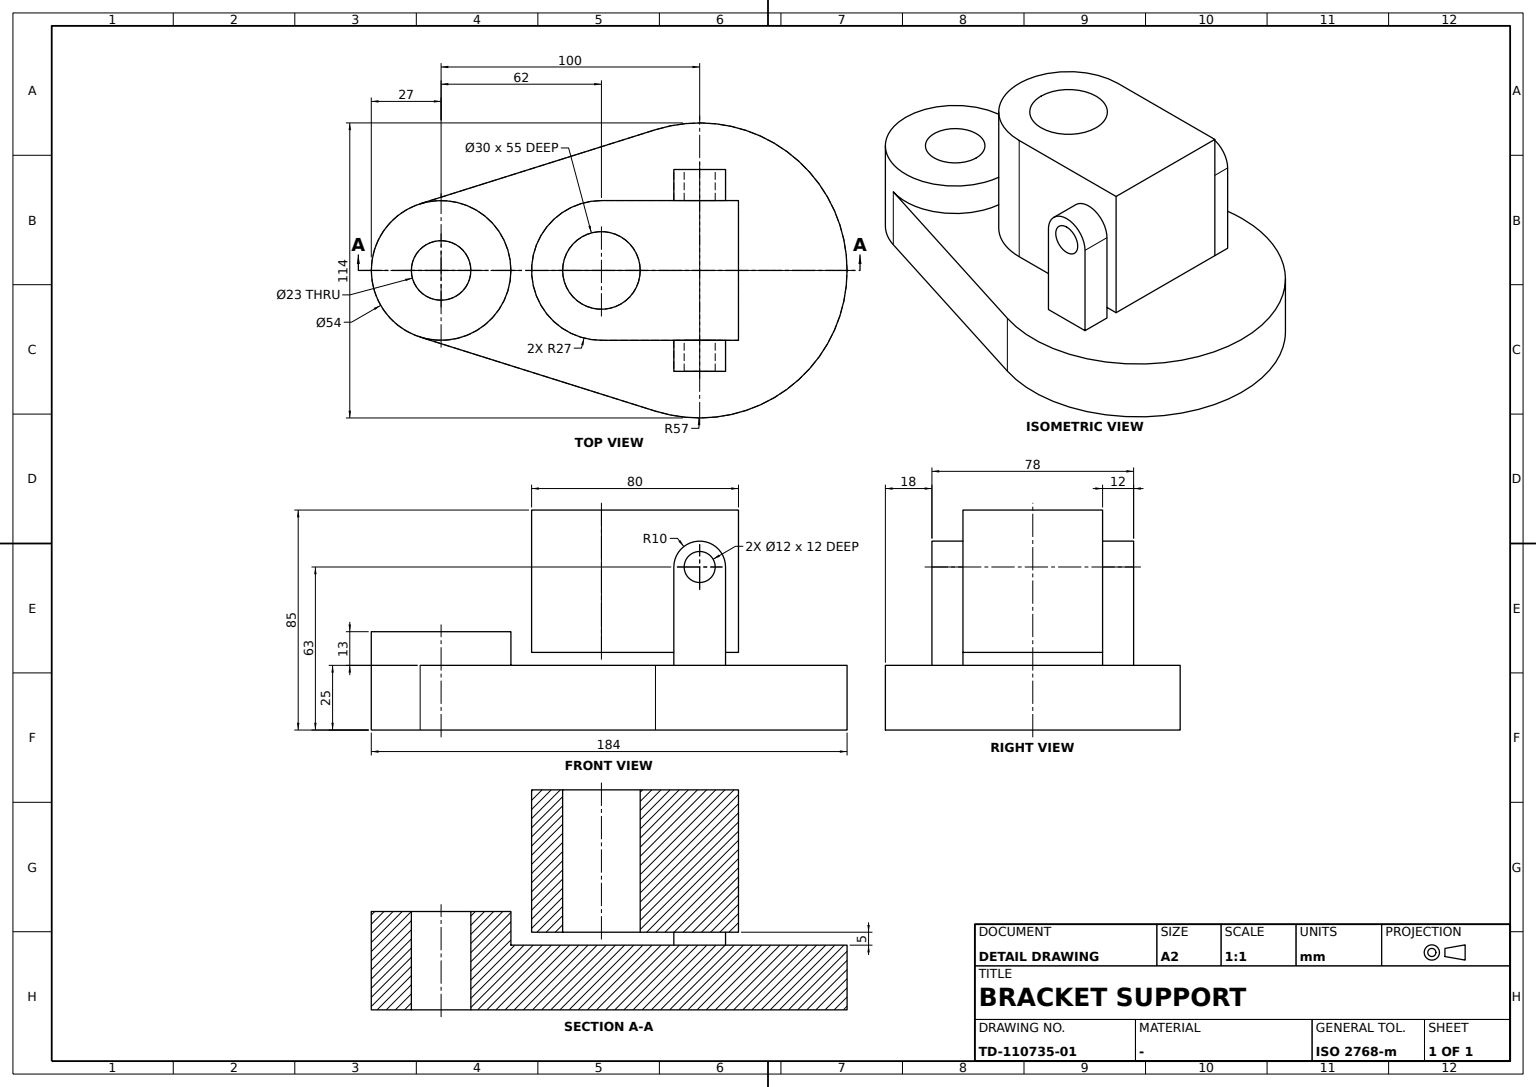
ISO-10303-21;
HEADER;
FILE_DESCRIPTION((''),'2;1');
FILE_NAME('','',(''),(''),'','','');
FILE_SCHEMA(('AUTOMOTIVE_DESIGN'));
ENDSEC;
DATA;
#1=APPLICATION_CONTEXT('');
#2=PRODUCT_CONTEXT('',#1,'mechanical');
#3=PRODUCT('','','',(#2));
#4=PRODUCT_DEFINITION_FORMATION('','',#3);
#5=PRODUCT_DEFINITION_CONTEXT('',#1,'design');
#6=PRODUCT_DEFINITION('','',#4,#5);
#7=PRODUCT_DEFINITION_SHAPE('','',#6);
#8=(LENGTH_UNIT()NAMED_UNIT(*)SI_UNIT(.MILLI.,.METRE.));
#9=(NAMED_UNIT(*)PLANE_ANGLE_UNIT()SI_UNIT($,.RADIAN.));
#10=(NAMED_UNIT(*)SI_UNIT($,.STERADIAN.)SOLID_ANGLE_UNIT());
#11=UNCERTAINTY_MEASURE_WITH_UNIT(LENGTH_MEASURE(0.005),#8,'distance_accuracy_value','');
#12=(GEOMETRIC_REPRESENTATION_CONTEXT(3)GLOBAL_UNCERTAINTY_ASSIGNED_CONTEXT((#11))GLOBAL_UNIT_ASSIGNED_CONTEXT((#8,#9,#10))REPRESENTATION_CONTEXT('',''));
#13=CARTESIAN_POINT('',(100.,27.,69.));
#14=VERTEX_POINT('',#13);
#15=CARTESIAN_POINT('',(100.,27.,63.));
#16=DIRECTION('',(0.,1.,0.));
#17=DIRECTION('',(0.,0.,1.));
#18=AXIS2_PLACEMENT_3D('',#15,#16,#17);
#19=CIRCLE('',#18,6.);
#20=EDGE_CURVE('',#14,#14,#19,.T.);
#21=ORIENTED_EDGE('',*,*,#20,.F.);
#22=EDGE_LOOP('',(#21));
#23=FACE_BOUND('',#22,.T.);
#24=CARTESIAN_POINT('',(100.,39.,57.));
#25=VERTEX_POINT('',#24);
#26=CARTESIAN_POINT('',(100.,39.,63.));
#27=DIRECTION('',(0.,-1.,0.));
#28=DIRECTION('',(0.,0.,-1.));
#29=AXIS2_PLACEMENT_3D('',#26,#27,#28);
#30=CIRCLE('',#29,6.);
#31=EDGE_CURVE('',#25,#25,#30,.F.);
#32=ORIENTED_EDGE('',*,*,#31,.T.);
#33=EDGE_LOOP('',(#32));
#34=FACE_BOUND('',#33,.T.);
#35=CARTESIAN_POINT('',(100.,-9.66,63.));
#36=DIRECTION('',(-1.,0.,0.));
#37=AXIS2_PLACEMENT_3D('',#35,#16,#36);
#38=CYLINDRICAL_SURFACE('',#37,6.);
#39=ADVANCED_FACE('',(#23,#34),#38,.F.);
#40=CARTESIAN_POINT('',(115.,-27.,85.));
#41=VERTEX_POINT('',#40);
#42=CARTESIAN_POINT('',(115.,27.,85.));
#43=VERTEX_POINT('',#42);
#44=CARTESIAN_POINT('',(115.,0.,85.));
#45=VECTOR('',#16,1000.);
#46=LINE('',#44,#45);
#47=EDGE_CURVE('',#41,#43,#46,.T.);
#48=ORIENTED_EDGE('',*,*,#47,.F.);
#49=CARTESIAN_POINT('',(115.,-27.,30.));
#50=VERTEX_POINT('',#49);
#51=CARTESIAN_POINT('',(115.,-27.,25.));
#52=VECTOR('',#17,1000.);
#53=LINE('',#51,#52);
#54=EDGE_CURVE('',#50,#41,#53,.T.);
#55=ORIENTED_EDGE('',*,*,#54,.F.);
#56=CARTESIAN_POINT('',(115.,27.,30.));
#57=VERTEX_POINT('',#56);
#58=CARTESIAN_POINT('',(115.,0.,30.));
#59=LINE('',#58,#45);
#60=EDGE_CURVE('',#50,#57,#59,.T.);
#61=ORIENTED_EDGE('',*,*,#60,.T.);
#62=CARTESIAN_POINT('',(115.,27.,25.));
#63=LINE('',#62,#52);
#64=EDGE_CURVE('',#57,#43,#63,.T.);
#65=ORIENTED_EDGE('',*,*,#64,.T.);
#66=EDGE_LOOP('',(#48,#55,#61,#65));
#67=FACE_BOUND('',#66,.T.);
#68=AXIS2_PLACEMENT_3D('',#58,#36,#17);
#69=PLANE('',#68);
#70=ADVANCED_FACE('',(#67),#69,.F.);
#71=CARTESIAN_POINT('',(100.,-39.,57.));
#72=VERTEX_POINT('',#71);
#73=CARTESIAN_POINT('',(100.,-39.,63.));
#74=AXIS2_PLACEMENT_3D('',#73,#27,#28);
#75=CIRCLE('',#74,6.);
#76=EDGE_CURVE('',#72,#72,#75,.T.);
#77=ORIENTED_EDGE('',*,*,#76,.F.);
#78=EDGE_LOOP('',(#77));
#79=FACE_BOUND('',#78,.T.);
#80=CARTESIAN_POINT('',(90.,-39.,25.));
#81=VERTEX_POINT('',#80);
#82=CARTESIAN_POINT('',(90.,-39.,63.));
#83=VERTEX_POINT('',#82);
#84=LINE('',#80,#52);
#85=EDGE_CURVE('',#81,#83,#84,.T.);
#86=ORIENTED_EDGE('',*,*,#85,.F.);
#87=CARTESIAN_POINT('',(110.,-39.,25.));
#88=VERTEX_POINT('',#87);
#89=CARTESIAN_POINT('',(0.,-39.,25.));
#90=DIRECTION('',(1.,0.,0.));
#91=VECTOR('',#90,1000.);
#92=LINE('',#89,#91);
#93=EDGE_CURVE('',#81,#88,#92,.T.);
#94=ORIENTED_EDGE('',*,*,#93,.T.);
#95=CARTESIAN_POINT('',(110.,-39.,62.999996));
#96=VERTEX_POINT('',#95);
#97=LINE('',#87,#52);
#98=EDGE_CURVE('',#88,#96,#97,.T.);
#99=ORIENTED_EDGE('',*,*,#98,.T.);
#100=CIRCLE('',#74,10.);
#101=EDGE_CURVE('',#96,#83,#100,.T.);
#102=ORIENTED_EDGE('',*,*,#101,.T.);
#103=EDGE_LOOP('',(#86,#94,#99,#102));
#104=FACE_BOUND('',#103,.T.);
#105=AXIS2_PLACEMENT_3D('',#80,#27,#90);
#106=PLANE('',#105);
#107=ADVANCED_FACE('',(#79,#104),#106,.T.);
#108=CARTESIAN_POINT('',(90.,-27.,25.));
#109=VERTEX_POINT('',#108);
#110=CARTESIAN_POINT('',(90.,-27.,30.));
#111=VERTEX_POINT('',#110);
#112=LINE('',#108,#52);
#113=EDGE_CURVE('',#109,#111,#112,.T.);
#114=ORIENTED_EDGE('',*,*,#113,.T.);
#115=CARTESIAN_POINT('',(110.,-27.,30.));
#116=VERTEX_POINT('',#115);
#117=LINE('',#115,#91);
#118=EDGE_CURVE('',#111,#116,#117,.T.);
#119=ORIENTED_EDGE('',*,*,#118,.T.);
#120=CARTESIAN_POINT('',(110.,-27.,25.));
#121=VERTEX_POINT('',#120);
#122=LINE('',#120,#52);
#123=EDGE_CURVE('',#121,#116,#122,.T.);
#124=ORIENTED_EDGE('',*,*,#123,.F.);
#125=CARTESIAN_POINT('',(0.,-27.,25.));
#126=VECTOR('',#36,1000.);
#127=LINE('',#125,#126);
#128=EDGE_CURVE('',#121,#109,#127,.T.);
#129=ORIENTED_EDGE('',*,*,#128,.T.);
#130=EDGE_LOOP('',(#114,#119,#124,#129));
#131=FACE_BOUND('',#130,.T.);
#132=AXIS2_PLACEMENT_3D('',#120,#16,#36);
#133=PLANE('',#132);
#134=ADVANCED_FACE('',(#131),#133,.T.);
#135=CARTESIAN_POINT('',(62.,27.,85.));
#136=VERTEX_POINT('',#135);
#137=CARTESIAN_POINT('',(62.,27.,30.));
#138=VERTEX_POINT('',#137);
#139=CARTESIAN_POINT('',(62.,27.,57.5));
#140=VECTOR('',#28,1000.);
#141=LINE('',#139,#140);
#142=EDGE_CURVE('',#136,#138,#141,.T.);
#143=ORIENTED_EDGE('',*,*,#142,.T.);
#144=CARTESIAN_POINT('',(62.,-27.,30.));
#145=VERTEX_POINT('',#144);
#146=CARTESIAN_POINT('',(62.,0.,30.));
#147=AXIS2_PLACEMENT_3D('',#146,#17,#90);
#148=CIRCLE('',#147,27.);
#149=EDGE_CURVE('',#138,#145,#148,.T.);
#150=ORIENTED_EDGE('',*,*,#149,.T.);
#151=CARTESIAN_POINT('',(62.,-27.,85.));
#152=VERTEX_POINT('',#151);
#153=CARTESIAN_POINT('',(62.,-27.,57.5));
#154=LINE('',#153,#140);
#155=EDGE_CURVE('',#152,#145,#154,.T.);
#156=ORIENTED_EDGE('',*,*,#155,.F.);
#157=CARTESIAN_POINT('',(62.,0.,85.));
#158=AXIS2_PLACEMENT_3D('',#157,#28,#36);
#159=CIRCLE('',#158,27.);
#160=EDGE_CURVE('',#152,#136,#159,.T.);
#161=ORIENTED_EDGE('',*,*,#160,.T.);
#162=EDGE_LOOP('',(#143,#150,#156,#161));
#163=FACE_BOUND('',#162,.T.);
#164=CARTESIAN_POINT('',(62.,0.,57.5));
#165=AXIS2_PLACEMENT_3D('',#164,#28,#27);
#166=CYLINDRICAL_SURFACE('',#165,27.);
#167=ADVANCED_FACE('',(#163),#166,.T.);
#168=CARTESIAN_POINT('',(47.,0.,85.));
#169=VERTEX_POINT('',#168);
#170=CIRCLE('',#158,15.);
#171=EDGE_CURVE('',#169,#169,#170,.T.);
#172=ORIENTED_EDGE('',*,*,#171,.T.);
#173=EDGE_LOOP('',(#172));
#174=FACE_BOUND('',#173,.T.);
#175=CARTESIAN_POINT('',(110.,-27.,85.));
#176=LINE('',#175,#126);
#177=EDGE_CURVE('',#41,#152,#176,.T.);
#178=ORIENTED_EDGE('',*,*,#177,.F.);
#179=ORIENTED_EDGE('',*,*,#47,.T.);
#180=CARTESIAN_POINT('',(110.,27.,85.));
#181=LINE('',#180,#126);
#182=EDGE_CURVE('',#43,#136,#181,.T.);
#183=ORIENTED_EDGE('',*,*,#182,.T.);
#184=ORIENTED_EDGE('',*,*,#160,.F.);
#185=EDGE_LOOP('',(#178,#179,#183,#184));
#186=FACE_BOUND('',#185,.T.);
#187=AXIS2_PLACEMENT_3D('',#44,#28,#36);
#188=PLANE('',#187);
#189=ADVANCED_FACE('',(#174,#186),#188,.F.);
#190=CARTESIAN_POINT('',(100.,-27.,69.));
#191=VERTEX_POINT('',#190);
#192=CARTESIAN_POINT('',(100.,-27.,63.));
#193=AXIS2_PLACEMENT_3D('',#192,#16,#17);
#194=CIRCLE('',#193,6.);
#195=EDGE_CURVE('',#191,#191,#194,.T.);
#196=ORIENTED_EDGE('',*,*,#195,.F.);
#197=EDGE_LOOP('',(#196));
#198=FACE_BOUND('',#197,.T.);
#199=ADVANCED_FACE('',(#198),#133,.F.);
#200=CARTESIAN_POINT('',(90.,27.,25.));
#201=VERTEX_POINT('',#200);
#202=CARTESIAN_POINT('',(90.,39.,25.));
#203=VERTEX_POINT('',#202);
#204=CARTESIAN_POINT('',(90.,0.,25.));
#205=LINE('',#204,#45);
#206=EDGE_CURVE('',#201,#203,#205,.T.);
#207=ORIENTED_EDGE('',*,*,#206,.F.);
#208=CARTESIAN_POINT('',(90.,27.,30.));
#209=VERTEX_POINT('',#208);
#210=LINE('',#200,#52);
#211=EDGE_CURVE('',#201,#209,#210,.T.);
#212=ORIENTED_EDGE('',*,*,#211,.T.);
#213=CARTESIAN_POINT('',(90.,27.,63.));
#214=VERTEX_POINT('',#213);
#215=EDGE_CURVE('',#209,#214,#210,.T.);
#216=ORIENTED_EDGE('',*,*,#215,.T.);
#217=CARTESIAN_POINT('',(90.,39.,63.));
#218=VERTEX_POINT('',#217);
#219=CARTESIAN_POINT('',(90.,33.,63.));
#220=LINE('',#219,#45);
#221=EDGE_CURVE('',#214,#218,#220,.T.);
#222=ORIENTED_EDGE('',*,*,#221,.T.);
#223=LINE('',#202,#52);
#224=EDGE_CURVE('',#203,#218,#223,.T.);
#225=ORIENTED_EDGE('',*,*,#224,.F.);
#226=EDGE_LOOP('',(#207,#212,#216,#222,#225));
#227=FACE_BOUND('',#226,.T.);
#228=AXIS2_PLACEMENT_3D('',#200,#90,#16);
#229=PLANE('',#228);
#230=ADVANCED_FACE('',(#227),#229,.F.);
#231=CARTESIAN_POINT('',(110.,27.,25.));
#232=VERTEX_POINT('',#231);
#233=CARTESIAN_POINT('',(110.,27.,30.));
#234=VERTEX_POINT('',#233);
#235=LINE('',#231,#52);
#236=EDGE_CURVE('',#232,#234,#235,.T.);
#237=ORIENTED_EDGE('',*,*,#236,.T.);
#238=LINE('',#233,#91);
#239=EDGE_CURVE('',#209,#234,#238,.T.);
#240=ORIENTED_EDGE('',*,*,#239,.F.);
#241=ORIENTED_EDGE('',*,*,#211,.F.);
#242=CARTESIAN_POINT('',(0.,27.,25.));
#243=LINE('',#242,#126);
#244=EDGE_CURVE('',#232,#201,#243,.T.);
#245=ORIENTED_EDGE('',*,*,#244,.F.);
#246=EDGE_LOOP('',(#237,#240,#241,#245));
#247=FACE_BOUND('',#246,.T.);
#248=AXIS2_PLACEMENT_3D('',#231,#16,#36);
#249=PLANE('',#248);
#250=ADVANCED_FACE('',(#247),#249,.F.);
#251=CARTESIAN_POINT('',(82.9,-54.374534,25.));
#252=VERTEX_POINT('',#251);
#253=CARTESIAN_POINT('',(82.9,54.374534,25.));
#254=VERTEX_POINT('',#253);
#255=CARTESIAN_POINT('',(100.,0.,25.));
#256=AXIS2_PLACEMENT_3D('',#255,#17,#90);
#257=CIRCLE('',#256,57.);
#258=EDGE_CURVE('',#252,#254,#257,.T.);
#259=ORIENTED_EDGE('',*,*,#258,.F.);
#260=CARTESIAN_POINT('',(82.9,-54.374534,0.));
#261=VERTEX_POINT('',#260);
#262=CARTESIAN_POINT('',(82.9,-54.374534,12.5));
#263=LINE('',#262,#52);
#264=EDGE_CURVE('',#261,#252,#263,.T.);
#265=ORIENTED_EDGE('',*,*,#264,.F.);
#266=CARTESIAN_POINT('',(82.9,54.374534,0.));
#267=VERTEX_POINT('',#266);
#268=CARTESIAN_POINT('',(100.,0.,0.));
#269=AXIS2_PLACEMENT_3D('',#268,#17,#90);
#270=CIRCLE('',#269,57.);
#271=EDGE_CURVE('',#261,#267,#270,.T.);
#272=ORIENTED_EDGE('',*,*,#271,.T.);
#273=CARTESIAN_POINT('',(82.9,54.374534,12.5));
#274=LINE('',#273,#52);
#275=EDGE_CURVE('',#267,#254,#274,.T.);
#276=ORIENTED_EDGE('',*,*,#275,.T.);
#277=EDGE_LOOP('',(#259,#265,#272,#276));
#278=FACE_BOUND('',#277,.T.);
#279=CARTESIAN_POINT('',(100.,0.,12.5));
#280=AXIS2_PLACEMENT_3D('',#279,#17,#90);
#281=CYLINDRICAL_SURFACE('',#280,57.);
#282=ADVANCED_FACE('',(#278),#281,.T.);
#283=CARTESIAN_POINT('',(90.,-27.,62.999996));
#284=VERTEX_POINT('',#283);
#285=CARTESIAN_POINT('',(110.,-27.,63.));
#286=VERTEX_POINT('',#285);
#287=CIRCLE('',#193,10.);
#288=EDGE_CURVE('',#284,#286,#287,.T.);
#289=ORIENTED_EDGE('',*,*,#288,.F.);
#290=EDGE_CURVE('',#83,#284,#220,.T.);
#291=ORIENTED_EDGE('',*,*,#290,.F.);
#292=ORIENTED_EDGE('',*,*,#101,.F.);
#293=CARTESIAN_POINT('',(110.,33.,63.));
#294=LINE('',#293,#45);
#295=EDGE_CURVE('',#96,#286,#294,.T.);
#296=ORIENTED_EDGE('',*,*,#295,.T.);
#297=EDGE_LOOP('',(#289,#291,#292,#296));
#298=FACE_BOUND('',#297,.T.);
#299=CARTESIAN_POINT('',(100.,33.,63.));
#300=AXIS2_PLACEMENT_3D('',#299,#16,#36);
#301=CYLINDRICAL_SURFACE('',#300,10.);
#302=ADVANCED_FACE('',(#298),#301,.T.);
#303=ORIENTED_EDGE('',*,*,#142,.F.);
#304=ORIENTED_EDGE('',*,*,#182,.F.);
#305=ORIENTED_EDGE('',*,*,#64,.F.);
#306=EDGE_CURVE('',#234,#57,#238,.T.);
#307=ORIENTED_EDGE('',*,*,#306,.F.);
#308=CARTESIAN_POINT('',(110.,27.,62.999996));
#309=VERTEX_POINT('',#308);
#310=EDGE_CURVE('',#234,#309,#235,.T.);
#311=ORIENTED_EDGE('',*,*,#310,.T.);
#312=CIRCLE('',#18,10.);
#313=EDGE_CURVE('',#214,#309,#312,.T.);
#314=ORIENTED_EDGE('',*,*,#313,.F.);
#315=ORIENTED_EDGE('',*,*,#215,.F.);
#316=EDGE_CURVE('',#138,#209,#238,.T.);
#317=ORIENTED_EDGE('',*,*,#316,.F.);
#318=EDGE_LOOP('',(#303,#304,#305,#307,#311,#314,#315,#317));
#319=FACE_BOUND('',#318,.T.);
#320=ADVANCED_FACE('',(#319),#249,.T.);
#321=ORIENTED_EDGE('',*,*,#288,.T.);
#322=EDGE_CURVE('',#116,#286,#122,.T.);
#323=ORIENTED_EDGE('',*,*,#322,.F.);
#324=EDGE_CURVE('',#116,#50,#117,.T.);
#325=ORIENTED_EDGE('',*,*,#324,.T.);
#326=ORIENTED_EDGE('',*,*,#54,.T.);
#327=ORIENTED_EDGE('',*,*,#177,.T.);
#328=ORIENTED_EDGE('',*,*,#155,.T.);
#329=EDGE_CURVE('',#145,#111,#117,.T.);
#330=ORIENTED_EDGE('',*,*,#329,.T.);
#331=EDGE_CURVE('',#111,#284,#112,.T.);
#332=ORIENTED_EDGE('',*,*,#331,.T.);
#333=EDGE_LOOP('',(#321,#323,#325,#326,#327,#328,#330,#332));
#334=FACE_BOUND('',#333,.T.);
#335=ADVANCED_FACE('',(#334),#133,.F.);
#336=ORIENTED_EDGE('',*,*,#20,.T.);
#337=EDGE_LOOP('',(#336));
#338=FACE_BOUND('',#337,.T.);
#339=ADVANCED_FACE('',(#338),#249,.T.);
#340=CARTESIAN_POINT('',(110.,39.,25.));
#341=VERTEX_POINT('',#340);
#342=CARTESIAN_POINT('',(110.,39.,63.));
#343=VERTEX_POINT('',#342);
#344=LINE('',#340,#52);
#345=EDGE_CURVE('',#341,#343,#344,.T.);
#346=ORIENTED_EDGE('',*,*,#345,.T.);
#347=EDGE_CURVE('',#309,#343,#294,.T.);
#348=ORIENTED_EDGE('',*,*,#347,.F.);
#349=ORIENTED_EDGE('',*,*,#310,.F.);
#350=ORIENTED_EDGE('',*,*,#236,.F.);
#351=CARTESIAN_POINT('',(110.,0.,25.));
#352=VECTOR('',#27,1000.);
#353=LINE('',#351,#352);
#354=EDGE_CURVE('',#341,#232,#353,.T.);
#355=ORIENTED_EDGE('',*,*,#354,.F.);
#356=EDGE_LOOP('',(#346,#348,#349,#350,#355));
#357=FACE_BOUND('',#356,.T.);
#358=AXIS2_PLACEMENT_3D('',#340,#36,#27);
#359=PLANE('',#358);
#360=ADVANCED_FACE('',(#357),#359,.F.);
#361=ORIENTED_EDGE('',*,*,#313,.T.);
#362=ORIENTED_EDGE('',*,*,#347,.T.);
#363=CIRCLE('',#29,10.);
#364=EDGE_CURVE('',#343,#218,#363,.T.);
#365=ORIENTED_EDGE('',*,*,#364,.T.);
#366=ORIENTED_EDGE('',*,*,#221,.F.);
#367=EDGE_LOOP('',(#361,#362,#365,#366));
#368=FACE_BOUND('',#367,.T.);
#369=ADVANCED_FACE('',(#368),#301,.T.);
#370=ORIENTED_EDGE('',*,*,#113,.F.);
#371=LINE('',#200,#352);
#372=EDGE_CURVE('',#109,#81,#371,.T.);
#373=ORIENTED_EDGE('',*,*,#372,.T.);
#374=ORIENTED_EDGE('',*,*,#85,.T.);
#375=ORIENTED_EDGE('',*,*,#290,.T.);
#376=ORIENTED_EDGE('',*,*,#331,.F.);
#377=EDGE_LOOP('',(#370,#373,#374,#375,#376));
#378=FACE_BOUND('',#377,.T.);
#379=ADVANCED_FACE('',(#378),#229,.F.);
#380=CARTESIAN_POINT('',(-8.1,-25.756358,25.));
#381=VERTEX_POINT('',#380);
#382=DIRECTION('',(0.953939201,-0.3,0.));
#383=VECTOR('',#382,1000.);
#384=LINE('',#380,#383);
#385=EDGE_CURVE('',#381,#252,#384,.T.);
#386=ORIENTED_EDGE('',*,*,#385,.T.);
#387=ORIENTED_EDGE('',*,*,#258,.T.);
#388=CARTESIAN_POINT('',(-8.1,25.756358,25.));
#389=VERTEX_POINT('',#388);
#390=DIRECTION('',(0.953939201,0.3,0.));
#391=VECTOR('',#390,1000.);
#392=LINE('',#388,#391);
#393=EDGE_CURVE('',#389,#254,#392,.T.);
#394=ORIENTED_EDGE('',*,*,#393,.F.);
#395=CARTESIAN_POINT('',(0.,0.,25.));
#396=AXIS2_PLACEMENT_3D('',#395,#17,#90);
#397=CIRCLE('',#396,27.);
#398=EDGE_CURVE('',#381,#389,#397,.T.);
#399=ORIENTED_EDGE('',*,*,#398,.F.);
#400=EDGE_LOOP('',(#386,#387,#394,#399));
#401=FACE_BOUND('',#400,.T.);
#402=ORIENTED_EDGE('',*,*,#372,.F.);
#403=ORIENTED_EDGE('',*,*,#128,.F.);
#404=LINE('',#340,#45);
#405=EDGE_CURVE('',#88,#121,#404,.T.);
#406=ORIENTED_EDGE('',*,*,#405,.F.);
#407=ORIENTED_EDGE('',*,*,#93,.F.);
#408=EDGE_LOOP('',(#402,#403,#406,#407));
#409=FACE_BOUND('',#408,.T.);
#410=ORIENTED_EDGE('',*,*,#354,.T.);
#411=ORIENTED_EDGE('',*,*,#244,.T.);
#412=ORIENTED_EDGE('',*,*,#206,.T.);
#413=CARTESIAN_POINT('',(0.,39.,25.));
#414=LINE('',#413,#91);
#415=EDGE_CURVE('',#203,#341,#414,.T.);
#416=ORIENTED_EDGE('',*,*,#415,.T.);
#417=EDGE_LOOP('',(#410,#411,#412,#416));
#418=FACE_BOUND('',#417,.T.);
#419=PLANE('',#396);
#420=ADVANCED_FACE('',(#401,#409,#418),#419,.T.);
#421=ORIENTED_EDGE('',*,*,#275,.F.);
#422=CARTESIAN_POINT('',(-8.1,25.756358,0.));
#423=VERTEX_POINT('',#422);
#424=LINE('',#422,#391);
#425=EDGE_CURVE('',#423,#267,#424,.T.);
#426=ORIENTED_EDGE('',*,*,#425,.F.);
#427=CARTESIAN_POINT('',(-8.1,25.756358,12.5));
#428=LINE('',#427,#52);
#429=EDGE_CURVE('',#423,#389,#428,.T.);
#430=ORIENTED_EDGE('',*,*,#429,.T.);
#431=ORIENTED_EDGE('',*,*,#393,.T.);
#432=EDGE_LOOP('',(#421,#426,#430,#431));
#433=FACE_BOUND('',#432,.T.);
#434=DIRECTION('',(0.3,-0.953939201,0.));
#435=AXIS2_PLACEMENT_3D('',#422,#434,#390);
#436=PLANE('',#435);
#437=ADVANCED_FACE('',(#433),#436,.F.);
#438=ORIENTED_EDGE('',*,*,#295,.F.);
#439=ORIENTED_EDGE('',*,*,#98,.F.);
#440=ORIENTED_EDGE('',*,*,#405,.T.);
#441=ORIENTED_EDGE('',*,*,#123,.T.);
#442=ORIENTED_EDGE('',*,*,#322,.T.);
#443=EDGE_LOOP('',(#438,#439,#440,#441,#442));
#444=FACE_BOUND('',#443,.T.);
#445=ADVANCED_FACE('',(#444),#359,.F.);
#446=CARTESIAN_POINT('',(77.,0.,30.));
#447=VERTEX_POINT('',#446);
#448=CIRCLE('',#147,15.);
#449=EDGE_CURVE('',#447,#447,#448,.T.);
#450=ORIENTED_EDGE('',*,*,#449,.T.);
#451=EDGE_LOOP('',(#450));
#452=FACE_BOUND('',#451,.T.);
#453=ORIENTED_EDGE('',*,*,#316,.T.);
#454=ORIENTED_EDGE('',*,*,#239,.T.);
#455=ORIENTED_EDGE('',*,*,#306,.T.);
#456=ORIENTED_EDGE('',*,*,#60,.F.);
#457=ORIENTED_EDGE('',*,*,#324,.F.);
#458=ORIENTED_EDGE('',*,*,#118,.F.);
#459=ORIENTED_EDGE('',*,*,#329,.F.);
#460=ORIENTED_EDGE('',*,*,#149,.F.);
#461=EDGE_LOOP('',(#453,#454,#455,#456,#457,#458,#459,#460));
#462=FACE_BOUND('',#461,.T.);
#463=CARTESIAN_POINT('',(35.,0.,30.));
#464=AXIS2_PLACEMENT_3D('',#463,#17,#90);
#465=PLANE('',#464);
#466=ADVANCED_FACE('',(#452,#462),#465,.F.);
#467=CARTESIAN_POINT('',(11.5,0.,0.));
#468=VERTEX_POINT('',#467);
#469=CARTESIAN_POINT('',(0.,0.,0.));
#470=AXIS2_PLACEMENT_3D('',#469,#17,#90);
#471=CIRCLE('',#470,11.5);
#472=EDGE_CURVE('',#468,#468,#471,.T.);
#473=ORIENTED_EDGE('',*,*,#472,.F.);
#474=EDGE_LOOP('',(#473));
#475=FACE_BOUND('',#474,.T.);
#476=CARTESIAN_POINT('',(11.5,0.,38.));
#477=VERTEX_POINT('',#476);
#478=CARTESIAN_POINT('',(0.,0.,38.));
#479=AXIS2_PLACEMENT_3D('',#478,#17,#90);
#480=CIRCLE('',#479,11.5);
#481=EDGE_CURVE('',#477,#477,#480,.T.);
#482=ORIENTED_EDGE('',*,*,#481,.T.);
#483=EDGE_LOOP('',(#482));
#484=FACE_BOUND('',#483,.T.);
#485=CARTESIAN_POINT('',(0.,0.,31.5));
#486=AXIS2_PLACEMENT_3D('',#485,#17,#90);
#487=CYLINDRICAL_SURFACE('',#486,11.5);
#488=ADVANCED_FACE('',(#475,#484),#487,.F.);
#489=ORIENTED_EDGE('',*,*,#472,.T.);
#490=EDGE_LOOP('',(#489));
#491=FACE_BOUND('',#490,.T.);
#492=CARTESIAN_POINT('',(-8.1,-25.756358,0.));
#493=VERTEX_POINT('',#492);
#494=LINE('',#492,#383);
#495=EDGE_CURVE('',#493,#261,#494,.T.);
#496=ORIENTED_EDGE('',*,*,#495,.F.);
#497=CIRCLE('',#470,27.);
#498=EDGE_CURVE('',#423,#493,#497,.T.);
#499=ORIENTED_EDGE('',*,*,#498,.F.);
#500=ORIENTED_EDGE('',*,*,#425,.T.);
#501=ORIENTED_EDGE('',*,*,#271,.F.);
#502=EDGE_LOOP('',(#496,#499,#500,#501));
#503=FACE_BOUND('',#502,.T.);
#504=PLANE('',#470);
#505=ADVANCED_FACE('',(#491,#503),#504,.F.);
#506=ORIENTED_EDGE('',*,*,#449,.F.);
#507=EDGE_LOOP('',(#506));
#508=FACE_BOUND('',#507,.T.);
#509=ORIENTED_EDGE('',*,*,#171,.F.);
#510=EDGE_LOOP('',(#509));
#511=FACE_BOUND('',#510,.T.);
#512=CARTESIAN_POINT('',(62.,0.,84.9));
#513=AXIS2_PLACEMENT_3D('',#512,#28,#90);
#514=CYLINDRICAL_SURFACE('',#513,15.);
#515=ADVANCED_FACE('',(#508,#511),#514,.F.);
#516=ORIENTED_EDGE('',*,*,#31,.F.);
#517=EDGE_LOOP('',(#516));
#518=FACE_BOUND('',#517,.T.);
#519=ORIENTED_EDGE('',*,*,#345,.F.);
#520=ORIENTED_EDGE('',*,*,#415,.F.);
#521=ORIENTED_EDGE('',*,*,#224,.T.);
#522=ORIENTED_EDGE('',*,*,#364,.F.);
#523=EDGE_LOOP('',(#519,#520,#521,#522));
#524=FACE_BOUND('',#523,.T.);
#525=AXIS2_PLACEMENT_3D('',#202,#27,#90);
#526=PLANE('',#525);
#527=ADVANCED_FACE('',(#518,#524),#526,.F.);
#528=ORIENTED_EDGE('',*,*,#498,.T.);
#529=CARTESIAN_POINT('',(-8.1,-25.756358,12.5));
#530=LINE('',#529,#52);
#531=EDGE_CURVE('',#493,#381,#530,.T.);
#532=ORIENTED_EDGE('',*,*,#531,.T.);
#533=ORIENTED_EDGE('',*,*,#398,.T.);
#534=ORIENTED_EDGE('',*,*,#429,.F.);
#535=EDGE_LOOP('',(#528,#532,#533,#534));
#536=FACE_BOUND('',#535,.T.);
#537=CARTESIAN_POINT('',(27.,0.,38.));
#538=VERTEX_POINT('',#537);
#539=CIRCLE('',#479,27.);
#540=EDGE_CURVE('',#538,#538,#539,.T.);
#541=ORIENTED_EDGE('',*,*,#540,.F.);
#542=EDGE_LOOP('',(#541));
#543=FACE_BOUND('',#542,.T.);
#544=CARTESIAN_POINT('',(0.,0.,12.5));
#545=AXIS2_PLACEMENT_3D('',#544,#17,#90);
#546=CYLINDRICAL_SURFACE('',#545,27.);
#547=ADVANCED_FACE('',(#536,#543),#546,.T.);
#548=ORIENTED_EDGE('',*,*,#481,.F.);
#549=EDGE_LOOP('',(#548));
#550=FACE_BOUND('',#549,.T.);
#551=ORIENTED_EDGE('',*,*,#540,.T.);
#552=EDGE_LOOP('',(#551));
#553=FACE_BOUND('',#552,.T.);
#554=PLANE('',#479);
#555=ADVANCED_FACE('',(#550,#553),#554,.T.);
#556=ORIENTED_EDGE('',*,*,#195,.T.);
#557=EDGE_LOOP('',(#556));
#558=FACE_BOUND('',#557,.T.);
#559=ORIENTED_EDGE('',*,*,#76,.T.);
#560=EDGE_LOOP('',(#559));
#561=FACE_BOUND('',#560,.T.);
#562=ADVANCED_FACE('',(#558,#561),#38,.F.);
#563=ORIENTED_EDGE('',*,*,#495,.T.);
#564=ORIENTED_EDGE('',*,*,#264,.T.);
#565=ORIENTED_EDGE('',*,*,#385,.F.);
#566=ORIENTED_EDGE('',*,*,#531,.F.);
#567=EDGE_LOOP('',(#563,#564,#565,#566));
#568=FACE_BOUND('',#567,.T.);
#569=DIRECTION('',(-0.3,-0.953939201,0.));
#570=AXIS2_PLACEMENT_3D('',#492,#569,#382);
#571=PLANE('',#570);
#572=ADVANCED_FACE('',(#568),#571,.T.);
#573=CLOSED_SHELL('',(#39,#70,#107,#134,#167,#189,#199,#230,#250,#282,#302,#320,#335,#339,#360,#369,#379,#420,#437,#445,#466,#488,#505,#515,#527,#547,#555,#562,#572));
#574=MANIFOLD_SOLID_BREP('',#573);
#575=ADVANCED_BREP_SHAPE_REPRESENTATION('',(#574),#12);
#576=SHAPE_DEFINITION_REPRESENTATION(#7,#575);
ENDSEC;
END-ISO-10303-21;
